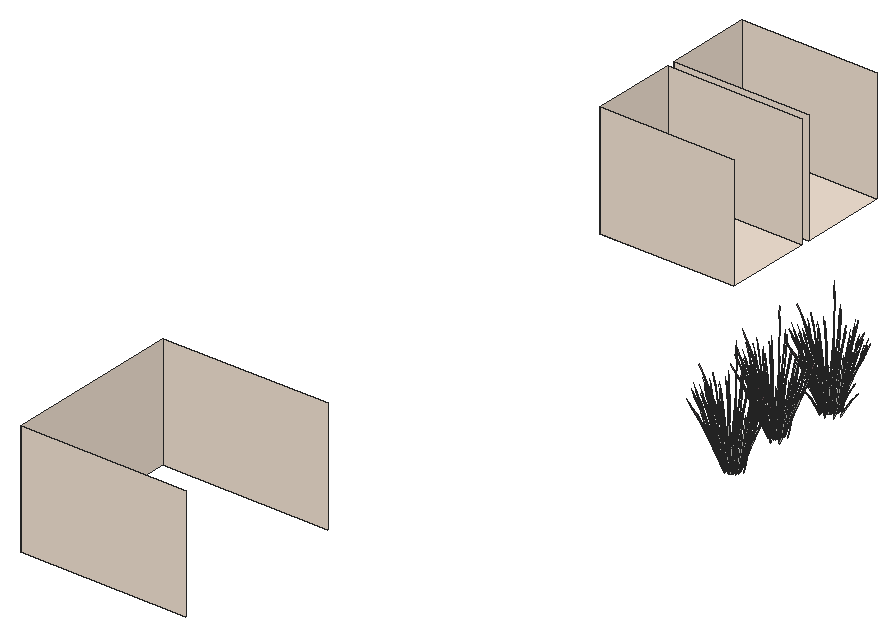
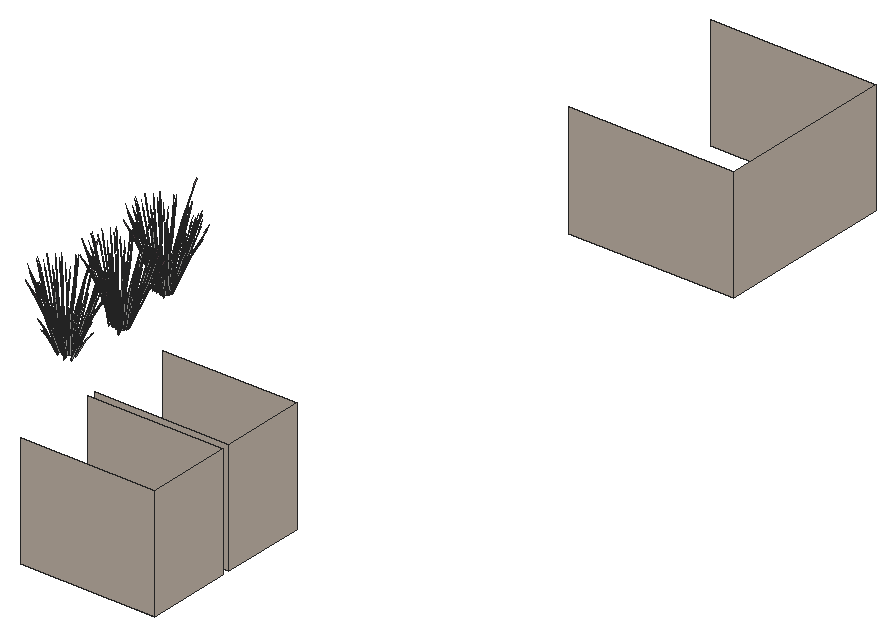
# SketchUp Ruby script. Lengths in inches.
U = 1.inch
M = Sketchup.active_model
def pt(a) = Geom::Point3d.new(a.map { |v| v * U })
def face(e, loops, mat)
  f = e.add_face(loops[0].map { |a| pt(a) })
  loops[1..].each { |l| e.add_face(l.map { |a| pt(a) }).erase! }
  f.material = f.back_material = mat if mat
  f
end
# faces: each face lists its corners as indices into pts; further lists are holes
def faces(e, pts, list, mat = nil) = list.each { |f| face(e, (f[0].is_a?(Array) ? f : [f]).map { |l| l.map { |i| pts[i] } }, mat) }
# xy, xz, yz: faces in a plane at the given z, y or x. An outline is a flat list of corners, or four numbers for a rectangle; further outlines are holes
def ring(l) = l.size == 4 ? [[l[0], l[1]], [l[2], l[1]], [l[2], l[3]], [l[0], l[3]]] : l.each_slice(2).to_a
def flat(e, list, mat, &to3) = list.each { |f| face(e, (f[0].is_a?(Array) ? f : [f]).map { |l| ring(l).map { |u, v| to3.(u, v) } }, mat) }
def xy(e, z, list, mat = nil) = flat(e, list, mat) { |x, y| [x, y, z] }
def xz(e, y, list, mat = nil) = flat(e, list, mat) { |x, z| [x, y, z] }
def yz(e, x, list, mat = nil) = flat(e, list, mat) { |y, z| [x, y, z] }
def lines(e, pts, list) = list.each { |a, b| e.add_line(pt(pts[a]), pt(pts[b])) }
# prism: a flat outline (further loops are holes) pulled along v
def prism(e, loops, v, mat = nil)
  f = face(e, loops, mat); d = Geom::Vector3d.new(v.map { |x| x * U })
  f.pushpull(f.normal.samedirection?(d) ? d.length : -d.length)
end
def box(e, o, s, mat = nil) = prism(e, [[o, [o[0] + s[0], o[1], o[2]], [o[0] + s[0], o[1] + s[1], o[2]], [o[0], o[1] + s[1], o[2]]]], [0, 0, s[2]], mat)
def at(x, y, z, deg = 0) = Geom::Transformation.translation(pt([x, y, z])) * Geom::Transformation.rotation(ORIGIN, Z_AXIS, deg.degrees)
def axes(o, x, y, z) = Geom::Transformation.new([*x, 0, *y, 0, *z, 0, *pt(o).to_a, 1])
def part(name) = M.definitions.add(name)
# library, detail: a bought-in or finely detailed component or shape, given as its bounding box
def library(name, o, s) = part(name).tap { |d| box(d.entities, o, s) }
def detail(e, o, s) = box(e.add_group.entities, o, s)
def put(e, d, t, mat = nil) = e.add_instance(d, t).tap { |i| i.material = mat if mat }
def group(e, t, mat = nil) = e.add_group.tap { |g| g.transformation = t; g.material = mat if mat }.entities
root = M.entities
M.materials.add("C01_Vanilla_Cream").color = [244, 228, 212]
M.materials.add("LightPink_Translucent").color = [144, 107, 117]
M.materials["LightPink_Translucent"].alpha = 0.75
c1 = part("blade")
p = [[2.15,0.21,22],[0,0.17,0],[0.09,0.45,0],[2.18,0.31,22],[2.29,0.31,22],[0.38,0.45,0],
  [2.48,0.24,33],[2.49,0.24,33],[2.48,0.22,33]]
faces(c1.entities,p,[[0,1,2,3],[4,5,2,3],[6,3,4,7],[8,0,3,6]])
c2 = part("seeds")
p = [[0.3,-0.1,1.38],[-0.01,-0.03,1.59],[-0.01,-0.03,0.03],[0.14,-0.07,-0.07],[0.29,-0.03,3],[0.15,0.01,3.11]]
faces(c2.entities,p,[[0,1,2,3],[1,0,4,5]],"LightPink_Translucent")
c3 = part("blade with seeds")
put(c3.entities,c1,at(0,0,0))
put(c3.entities,c2,axes([2.4,0.25,30.99],[1.5799,-0.05474,1.17369],[-0.12525,1.92788,0.29478],[-0.07173,-0.02425,1.56792]))
xy(root,501,[[240,327,290,358.5],[240,361.5,290,393]],"C01_Vanilla_Cream")
xz(root,75,[[226.53,501,288,543]],"C01_Vanilla_Cream")
xz(root,141,[[226.53,501,288,543]],"C01_Vanilla_Cream")
xz(root,327,[[240,501,290,543]],"C01_Vanilla_Cream")
xz(root,358.5,[[240,501,290,543]],"C01_Vanilla_Cream")
xz(root,361.5,[[240,501,290,543]],"C01_Vanilla_Cream")
xz(root,393,[[240,501,290,543]],"C01_Vanilla_Cream")
yz(root,226.53,[[75,501,141,543]],"C01_Vanilla_Cream")
yz(root,240,[[327,501,358.5,543],[361.5,501,393,543]],"C01_Vanilla_Cream")
put(root,c3,axes([353.4,268.07,500.07],[-0.01441,-0.29294,0.86145],[0.36003,0.20894,0.63294],[-0.07081,0.13963,0.18974]))
put(root,c3,axes([357.67,263.51,500.07],[-0.18544,0.25079,0.86145],[-0.15939,-0.33694,0.63294],[0.15316,-0.08443,0.18974]))
put(root,c3,axes([355.34,262.26,500.07],[0.07142,0.28728,0.86145],[-0.3962,-0.15911,0.63294],[0.04263,-0.1471,0.18974]))
put(root,c3,axes([354.97,286.16,500.07],[0.35544,-0.03525,0.86145],[-0.22547,0.31061,0.63294],[-0.17565,-0.04659,0.18974]))
put(root,c3,axes([359.68,288.375,500.07],[-0.31347,-0.14166,0.86145],[0.40476,-0.14393,0.63294],[0.10917,0.12192,0.18974]))
put(root,c3,axes([354.47,288.61,500.07],[0.23202,-0.22328,0.86145],[0.09155,0.35348,0.63294],[-0.16768,0.06329,0.18974]))
put(root,c3,axes([361.59,287.21,500.07],[-0.34399,0.08133,0.86145],[0.16192,-0.33614,0.63294],[0.18249,0.023,0.18974]))
put(root,c3,axes([356.34,284.13,500.07],[0.29042,0.17147,0.86145],[-0.42295,0.10307,0.63294],[-0.0905,-0.13178,0.18974]))
put(root,c3,axes([356.4375,289.59,500.07],[-0.01441,-0.29294,0.86145],[0.36003,0.20894,0.63294],[-0.07081,0.13963,0.18974]))
put(root,c3,axes([360.71,285.03,500.07],[-0.18544,0.25079,0.86145],[-0.15939,-0.33694,0.63294],[0.15316,-0.08443,0.18974]))
put(root,c3,axes([358.37,283.78,500.07],[0.07142,0.28728,0.86145],[-0.3962,-0.15911,0.63294],[0.04263,-0.1471,0.18974]))
put(root,c3,axes([358.92,241.3,500.13],[-0.01521,-0.46386,1.05954],[0.68831,0.12024,0.44862],[-0.1628,0.25382,1.00012]))
put(root,c3,axes([355.88,265.26,500.13],[-0.01521,-0.46386,1.05954],[0.68831,0.12024,0.44862],[-0.1628,0.25382,1.00012]))
put(root,c3,axes([358.92,286.78,500.13],[-0.01521,-0.46386,1.05954],[0.68831,0.12024,0.44862],[-0.1628,0.25382,1.00012]))
put(root,c3,axes([357.04,239.55,501.74],[-0.47473,-0.23813,-0.53284],[0.33738,-0.41728,0.0643],[-0.172,-0.14218,0.75375]))
put(root,c3,axes([357.55,243.21,501.74],[0.26572,0.40059,-0.53284],[-0.54698,0.22325,0.0643],[0.06214,0.19355,0.75375]))
put(root,c3,axes([356.07,240.14,501.74],[-0.55654,-0.01186,-0.53284],[0.03738,-0.49951,0.0643],[-0.23578,-0.05271,0.75375]))
put(root,c3,axes([360.06,240.62,501.74],[0.29081,-0.38873,-0.53284],[0.5096,0.27626,0.0643],[0.17364,-0.14084,0.75375]))
put(root,c3,axes([360.2,241.6,501.74],[0.48922,-0.21758,-0.53284],[0.27264,0.44789,0.0643],[0.23638,-0.05088,0.75375]))
put(root,c3,axes([359.34,239.83,501.74],[0.01449,-0.45571,-0.53284],[0.61002,0.03061,0.0643],[0.06438,-0.19306,0.75375]))
put(root,c3,axes([359.72,242.51,501.74],[0.55654,0.01186,-0.53284],[-0.03738,0.49951,0.0643],[0.23578,0.05271,0.75375]))
put(root,c3,axes([358.23,239.4375,501.74],[-0.26572,-0.40059,-0.53284],[0.54698,-0.22325,0.0643],[-0.06214,-0.19355,0.75375]))
put(root,c3,axes([354,263.52,501.74],[-0.47473,-0.23813,-0.53284],[0.33738,-0.41728,0.0643],[-0.172,-0.14218,0.75375]))
put(root,c3,axes([354.52,267.18,501.74],[0.26572,0.40059,-0.53284],[-0.54698,0.22325,0.0643],[0.06214,0.19355,0.75375]))
put(root,c3,axes([353.03,264.11,501.74],[-0.55654,-0.01186,-0.53284],[0.03738,-0.49951,0.0643],[-0.23578,-0.05271,0.75375]))
put(root,c3,axes([357.02,264.59,501.74],[0.29081,-0.38873,-0.53284],[0.5096,0.27626,0.0643],[0.17364,-0.14084,0.75375]))
put(root,c3,axes([357.16,265.57,501.74],[0.48922,-0.21758,-0.53284],[0.27264,0.44789,0.0643],[0.23638,-0.05088,0.75375]))
put(root,c3,axes([356.3,263.8,501.74],[0.01449,-0.45571,-0.53284],[0.61002,0.03061,0.0643],[0.06438,-0.19306,0.75375]))
put(root,c3,axes([356.68,266.48,501.74],[0.55654,0.01186,-0.53284],[-0.03738,0.49951,0.0643],[0.23578,0.05271,0.75375]))
put(root,c3,axes([355.2,263.4,501.74],[-0.26572,-0.40059,-0.53284],[0.54698,-0.22325,0.0643],[-0.06214,-0.19355,0.75375]))
put(root,c3,axes([357.04,285.04,501.74],[-0.47473,-0.23813,-0.53284],[0.33738,-0.41728,0.0643],[-0.172,-0.14218,0.75375]))
put(root,c3,axes([357.55,288.7,501.74],[0.26572,0.40059,-0.53284],[-0.54698,0.22325,0.0643],[0.06214,0.19355,0.75375]))
put(root,c3,axes([356.07,285.625,501.74],[-0.55654,-0.01186,-0.53284],[0.03738,-0.49951,0.0643],[-0.23578,-0.05271,0.75375]))
put(root,c3,axes([360.06,286.11,501.74],[0.29081,-0.38873,-0.53284],[0.5096,0.27626,0.0643],[0.17364,-0.14084,0.75375]))
put(root,c3,axes([360.2,287.09,501.74],[0.48922,-0.21758,-0.53284],[0.27264,0.44789,0.0643],[0.23638,-0.05088,0.75375]))
put(root,c3,axes([359.34,285.31,501.74],[0.01449,-0.45571,-0.53284],[0.61002,0.03061,0.0643],[0.06438,-0.19306,0.75375]))
put(root,c3,axes([359.72,287.99,501.74],[0.55654,0.01186,-0.53284],[-0.03738,0.49951,0.0643],[0.23578,0.05271,0.75375]))
put(root,c3,axes([358.23,284.92,501.74],[-0.26572,-0.40059,-0.53284],[0.54698,-0.22325,0.0643],[-0.06214,-0.19355,0.75375]))
put(root,c3,axes([357.75,243.29,501.51],[0.54728,0.1235,-0.38324],[-0.18759,0.42344,-0.29685],[0.05018,0.17048,0.7333]))
put(root,c3,axes([359.22,239.68,501.51],[-0.39855,-0.33102,-0.38324],[0.42102,-0.2899,-0.29685],[0.06064,-0.16819,0.7333]))
put(root,c3,axes([356.81,239.5625,501.51],[-0.54938,0.11711,-0.38324],[-0.0961,-0.44351,-0.29685],[-0.14756,-0.1271,0.7333]))
put(root,c3,axes([360.3,241.4375,501.51],[0.15083,-0.44814,-0.38324],[0.51712,0.15361,-0.29685],[0.2082,-0.04109,0.7333]))
put(root,c3,axes([355.88,240.24,501.51],[-0.40426,0.32635,-0.38324],[-0.35404,-0.34474,-0.29685],[-0.2054,-0.04965,0.7333]))
put(root,c3,axes([355.74,242.21,501.51],[0.14302,0.44985,-0.38324],[-0.54163,0.07869,-0.29685],[-0.15522,0.12083,0.7333]))
put(root,c3,axes([355.49,241.21,501.51],[-0.15083,0.44814,-0.38324],[-0.51712,-0.15361,-0.29685],[-0.2082,0.04109,0.7333]))
put(root,c3,axes([358.03,239.36,501.51],[-0.54728,-0.1235,-0.38324],[0.18759,-0.42344,-0.29685],[-0.05018,-0.17048,0.7333]))
put(root,c3,axes([360.04,240.44,501.51],[-0.14302,-0.44985,-0.38324],[0.54163,-0.07869,-0.29685],[0.15522,-0.12083,0.7333]))
put(root,c3,axes([358.97,243.09,501.51],[0.54938,-0.11711,-0.38324],[0.0961,0.44351,-0.29685],[0.14756,0.1271,0.7333]))
put(root,c3,axes([354.72,267.26,501.51],[0.54728,0.1235,-0.38324],[-0.18759,0.42344,-0.29685],[0.05018,0.17048,0.7333]))
put(root,c3,axes([356.18,263.65,501.51],[-0.39855,-0.33102,-0.38324],[0.42102,-0.2899,-0.29685],[0.06064,-0.16819,0.7333]))
put(root,c3,axes([353.78,263.53,501.51],[-0.54938,0.11711,-0.38324],[-0.0961,-0.44351,-0.29685],[-0.14756,-0.1271,0.7333]))
put(root,c3,axes([357.26,265.41,501.51],[0.15083,-0.44814,-0.38324],[0.51712,0.15361,-0.29685],[0.2082,-0.04109,0.7333]))
put(root,c3,axes([352.85,264.21,501.51],[-0.40426,0.32635,-0.38324],[-0.35404,-0.34474,-0.29685],[-0.2054,-0.04965,0.7333]))
put(root,c3,axes([352.71,266.17,501.51],[0.14302,0.44985,-0.38324],[-0.54163,0.07869,-0.29685],[-0.15522,0.12083,0.7333]))
put(root,c3,axes([352.45,265.18,501.51],[-0.15083,0.44814,-0.38324],[-0.51712,-0.15361,-0.29685],[-0.2082,0.04109,0.7333]))
put(root,c3,axes([355,263.32,501.51],[-0.54728,-0.1235,-0.38324],[0.18759,-0.42344,-0.29685],[-0.05018,-0.17048,0.7333]))
put(root,c3,axes([357.01,264.41,501.51],[-0.14302,-0.44985,-0.38324],[0.54163,-0.07869,-0.29685],[0.15522,-0.12083,0.7333]))
put(root,c3,axes([355.9375,267.05,501.51],[0.54938,-0.11711,-0.38324],[0.0961,0.44351,-0.29685],[0.14756,0.1271,0.7333]))
put(root,c3,axes([357.75,288.78,501.51],[0.54728,0.1235,-0.38324],[-0.18759,0.42344,-0.29685],[0.05018,0.17048,0.7333]))
put(root,c3,axes([359.22,285.16,501.51],[-0.39855,-0.33102,-0.38324],[0.42102,-0.2899,-0.29685],[0.06064,-0.16819,0.7333]))
put(root,c3,axes([356.81,285.05,501.51],[-0.54938,0.11711,-0.38324],[-0.0961,-0.44351,-0.29685],[-0.14756,-0.1271,0.7333]))
put(root,c3,axes([360.3,286.92,501.51],[0.15083,-0.44814,-0.38324],[0.51712,0.15361,-0.29685],[0.2082,-0.04109,0.7333]))
put(root,c3,axes([355.88,285.73,501.51],[-0.40426,0.32635,-0.38324],[-0.35404,-0.34474,-0.29685],[-0.2054,-0.04965,0.7333]))
put(root,c3,axes([355.74,287.69,501.51],[0.14302,0.44985,-0.38324],[-0.54163,0.07869,-0.29685],[-0.15522,0.12083,0.7333]))
put(root,c3,axes([355.49,286.69,501.51],[-0.15083,0.44814,-0.38324],[-0.51712,-0.15361,-0.29685],[-0.2082,0.04109,0.7333]))
put(root,c3,axes([358.03,284.84,501.51],[-0.54728,-0.1235,-0.38324],[0.18759,-0.42344,-0.29685],[-0.05018,-0.17048,0.7333]))
put(root,c3,axes([360.04,285.93,501.51],[-0.14302,-0.44985,-0.38324],[0.54163,-0.07869,-0.29685],[0.15522,-0.12083,0.7333]))
put(root,c3,axes([358.97,288.57,501.51],[0.54938,-0.11711,-0.38324],[0.0961,0.44351,-0.29685],[0.14756,0.1271,0.7333]))
put(root,c3,axes([356.45,242.82,502],[-0.01449,0.45571,-0.59145],[-0.61002,-0.03061,0.07138],[-0.06438,0.19306,0.83667]))
put(root,c3,axes([353.41,266.79,502],[-0.01449,0.45571,-0.59145],[-0.61002,-0.03061,0.07138],[-0.06438,0.19306,0.83667]))
put(root,c3,axes([356.45,288.3,502],[-0.01449,0.45571,-0.59145],[-0.61002,-0.03061,0.07138],[-0.06438,0.19306,0.83667]))
put(root,c3,axes([356.57,242.97,501.75],[0.39855,0.33102,-0.4254],[-0.42102,0.2899,-0.32951],[-0.06064,0.16819,0.81396]))
put(root,c3,axes([353.53,266.9375,501.75],[0.39855,0.33102,-0.4254],[-0.42102,0.2899,-0.32951],[-0.06064,0.16819,0.81396]))
put(root,c3,axes([356.57,288.46,501.75],[0.39855,0.33102,-0.4254],[-0.42102,0.2899,-0.32951],[-0.06064,0.16819,0.81396]))
put(root,c3,axes([358.17,242.25,500.49],[0.48111,0.19866,1.13446],[-0.47133,0.42798,0.44862],[-0.21112,-0.25366,0.95105]))
put(root,c3,axes([355.14,266.21,500.49],[0.48111,0.19866,1.13446],[-0.47133,0.42798,0.44862],[-0.21112,-0.25366,0.95105]))
put(root,c3,axes([358.17,287.73,500.49],[0.48111,0.19866,1.13446],[-0.47133,0.42798,0.44862],[-0.21112,-0.25366,0.95105]))
put(root,c3,axes([356.58,240.9375,500.51],[0.15825,-0.07127,1.32798],[0.05457,0.4976,0.10393],[-0.34278,0.06603,0.47463]))
put(root,c3,axes([353.55,264.9,500.51],[0.15825,-0.07127,1.32798],[0.05457,0.4976,0.10393],[-0.34278,0.06603,0.47463]))
put(root,c3,axes([356.58,286.42,500.51],[0.15825,-0.07127,1.32798],[0.05457,0.4976,0.10393],[-0.34278,0.06603,0.47463]))
put(root,c3,axes([356.24,243.46,500.52],[0.01223,-0.25433,1.15759],[0.55017,0.13434,0.15997],[-0.04767,0.27105,0.54661]))
put(root,c3,axes([353.21,267.43,500.52],[0.01223,-0.25433,1.15759],[0.55017,0.13434,0.15997],[-0.04767,0.27105,0.54661]))
put(root,c3,axes([356.24,288.95,500.52],[0.01223,-0.25433,1.15759],[0.55017,0.13434,0.15997],[-0.04767,0.27105,0.54661]))
put(root,c3,axes([360.05,242.71,501.39],[0.31678,0.30846,-0.2656],[-0.36171,0.29199,0.3429],[0.18378,0.04443,0.65611]))
put(root,c3,axes([355.17,241.01,501.39],[-0.46269,-0.13744,-0.2656],[0.13495,-0.40096,0.3429],[-0.18628,0.03677,0.65611]))
put(root,c3,axes([355.34,242.16,501.39],[-0.48462,0.07041,-0.2656],[-0.12797,-0.4025,0.3429],[-0.13888,0.10811,0.65611]))
put(root,c3,axes([360.61,241.64,501.39],[0.46269,0.13744,-0.2656],[-0.13495,0.40096,0.3429],[0.18628,-0.03677,0.65611]))
put(root,c3,axes([356.87,239.24,501.39],[-0.08599,-0.39682,-0.2656],[0.49155,-0.10478,0.3429],[-0.13203,-0.11372,0.65611]))
put(root,c3,axes([356.2,243.09,501.39],[-0.3767,0.25939,-0.2656],[-0.3566,-0.29618,0.3429],[-0.05426,0.15048,0.65611]))
put(root,c3,axes([360.44,240.49,501.39],[0.48462,-0.07041,-0.2656],[0.12797,0.4025,0.3429],[0.13888,-0.10811,0.65611]))
put(root,c3,axes([357.5,243.55,501.39],[-0.16784,0.37886,-0.2656],[-0.48968,-0.1105,0.3429],[0.0449,0.15254,0.65611]))
put(root,c3,axes([359.59,239.56,501.39],[0.3767,-0.25939,-0.2656],[0.3566,0.29618,0.3429],[0.05426,-0.15048,0.65611]))
put(root,c3,axes([358.28,239.1,501.39],[0.16784,-0.37886,-0.2656],[0.48968,0.1105,0.3429],[-0.0449,-0.15254,0.65611]))
put(root,c3,axes([355.73,239.93,501.39],[-0.31678,-0.30846,-0.2656],[0.36171,-0.29199,0.3429],[-0.18378,-0.04443,0.65611]))
put(root,c3,axes([357.02,266.68,501.39],[0.31678,0.30846,-0.2656],[-0.36171,0.29199,0.3429],[0.18378,0.04443,0.65611]))
put(root,c3,axes([352.14,264.97,501.39],[-0.46269,-0.13744,-0.2656],[0.13495,-0.40096,0.3429],[-0.18628,0.03677,0.65611]))
put(root,c3,axes([352.31,266.13,501.39],[-0.48462,0.07041,-0.2656],[-0.12797,-0.4025,0.3429],[-0.13888,0.10811,0.65611]))
put(root,c3,axes([357.58,265.61,501.39],[0.46269,0.13744,-0.2656],[-0.13495,0.40096,0.3429],[0.18628,-0.03677,0.65611]))
put(root,c3,axes([353.83,263.2,501.39],[-0.08599,-0.39682,-0.2656],[0.49155,-0.10478,0.3429],[-0.13203,-0.11372,0.65611]))
put(root,c3,axes([353.16,267.06,501.39],[-0.3767,0.25939,-0.2656],[-0.3566,-0.29618,0.3429],[-0.05426,0.15048,0.65611]))
put(root,c3,axes([357.41,264.45,501.39],[0.48462,-0.07041,-0.2656],[0.12797,0.4025,0.3429],[0.13888,-0.10811,0.65611]))
put(root,c3,axes([354.47,267.52,501.39],[-0.16784,0.37886,-0.2656],[-0.48968,-0.1105,0.3429],[0.0449,0.15254,0.65611]))
put(root,c3,axes([356.55,263.52,501.39],[0.3767,-0.25939,-0.2656],[0.3566,0.29618,0.3429],[0.05426,-0.15048,0.65611]))
put(root,c3,axes([355.25,263.0625,501.39],[0.16784,-0.37886,-0.2656],[0.48968,0.1105,0.3429],[-0.0449,-0.15254,0.65611]))
put(root,c3,axes([352.7,263.9,501.39],[-0.31678,-0.30846,-0.2656],[0.36171,-0.29199,0.3429],[-0.18378,-0.04443,0.65611]))
put(root,c3,axes([360.05,288.2,501.39],[0.31678,0.30846,-0.2656],[-0.36171,0.29199,0.3429],[0.18378,0.04443,0.65611]))
put(root,c3,axes([355.17,286.49,501.39],[-0.46269,-0.13744,-0.2656],[0.13495,-0.40096,0.3429],[-0.18628,0.03677,0.65611]))
put(root,c3,axes([355.34,287.65,501.39],[-0.48462,0.07041,-0.2656],[-0.12797,-0.4025,0.3429],[-0.13888,0.10811,0.65611]))
put(root,c3,axes([360.61,287.13,501.39],[0.46269,0.13744,-0.2656],[-0.13495,0.40096,0.3429],[0.18628,-0.03677,0.65611]))
put(root,c3,axes([356.87,284.72,501.39],[-0.08599,-0.39682,-0.2656],[0.49155,-0.10478,0.3429],[-0.13203,-0.11372,0.65611]))
put(root,c3,axes([356.2,288.58,501.39],[-0.3767,0.25939,-0.2656],[-0.3566,-0.29618,0.3429],[-0.05426,0.15048,0.65611]))
put(root,c3,axes([360.44,285.97,501.39],[0.48462,-0.07041,-0.2656],[0.12797,0.4025,0.3429],[0.13888,-0.10811,0.65611]))
put(root,c3,axes([357.5,289.04,501.39],[-0.16784,0.37886,-0.2656],[-0.48968,-0.1105,0.3429],[0.0449,0.15254,0.65611]))
put(root,c3,axes([359.59,285.04,501.39],[0.3767,-0.25939,-0.2656],[0.3566,0.29618,0.3429],[0.05426,-0.15048,0.65611]))
put(root,c3,axes([358.28,284.58,501.39],[0.16784,-0.37886,-0.2656],[0.48968,0.1105,0.3429],[-0.0449,-0.15254,0.65611]))
put(root,c3,axes([355.73,285.42,501.39],[-0.31678,-0.30846,-0.2656],[0.36171,-0.29199,0.3429],[-0.18378,-0.04443,0.65611]))
put(root,c3,axes([361,242.76,500.95],[-0.10656,-0.41414,-0.02619],[0.50364,-0.09521,-0.11874],[0.10517,0.02626,0.39164]))
put(root,c3,axes([357.96,266.73,500.95],[-0.10656,-0.41414,-0.02619],[0.50364,-0.09521,-0.11874],[0.10517,0.02626,0.39164]))
put(root,c3,axes([361,288.25,500.95],[-0.10656,-0.41414,-0.02619],[0.50364,-0.09521,-0.11874],[0.10517,0.02626,0.39164]))
put(root,c3,axes([358.92,241.92,500.91],[-0.2068,-0.08488,1.28532],[0.42797,-0.35609,0.10393],[0.26673,0.16064,0.54946]))
put(root,c3,axes([358.65,239.6,500.91],[-0.10366,0.16934,1.28532],[-0.43488,-0.35044,0.10393],[0.19618,-0.21841,0.54946]))
put(root,c3,axes([359.35,241.15,500.91],[-0.23093,0.01116,1.28532],[0.15319,-0.4836,0.10393],[0.32909,0.02991,0.54946]))
put(root,c3,axes([358.0625,242.42,500.91],[-0.12726,-0.15818,1.28532],[0.58807,-0.13317,0.10393],[0.13291,0.24832,0.54946]))
put(root,c3,axes([357.02,242.5,500.91],[-0.01363,-0.18909,1.28532],[0.5906,0.12544,0.10393],[-0.03653,0.26947,0.54946]))
put(root,c3,axes([356.08,242.14,500.91],[0.10366,-0.16934,1.28532],[0.43488,0.35044,0.10393],[-0.19618,0.21841,0.54946]))
put(root,c3,axes([355.47,241.44,500.91],[0.19317,-0.10421,1.28532],[0.16263,0.48153,0.10393],[-0.30326,0.10883,0.54946]))
put(root,c3,axes([356.18,241.77,500.91],[0.13906,-0.15138,1.28532],[0.35111,0.40859,0.10393],[-0.24082,0.18608,0.54946]))
put(root,c3,axes([356.67,239.32,500.91],[0.12726,0.15818,1.28532],[-0.58807,0.13317,0.10393],[-0.13291,-0.24832,0.54946]))
put(root,c3,axes([355.81,239.8125,500.91],[0.2068,0.08488,1.28532],[-0.42797,0.35609,0.10393],[-0.26673,-0.16064,0.54946]))
put(root,c3,axes([355.38,240.59,500.91],[0.23093,-0.01116,1.28532],[-0.15319,0.4836,0.10393],[-0.32909,-0.02991,0.54946]))
put(root,c3,axes([355.88,265.89,500.91],[-0.2068,-0.08488,1.28532],[0.42797,-0.35609,0.10393],[0.26673,0.16064,0.54946]))
put(root,c3,axes([355.62,263.57,500.91],[-0.10366,0.16934,1.28532],[-0.43488,-0.35044,0.10393],[0.19618,-0.21841,0.54946]))
put(root,c3,axes([356.31,265.11,500.91],[-0.23093,0.01116,1.28532],[0.15319,-0.4836,0.10393],[0.32909,0.02991,0.54946]))
put(root,c3,axes([355.03,266.38,500.91],[-0.12726,-0.15818,1.28532],[0.58807,-0.13317,0.10393],[0.13291,0.24832,0.54946]))
put(root,c3,axes([353.99,266.46,500.91],[-0.01363,-0.18909,1.28532],[0.5906,0.12544,0.10393],[-0.03653,0.26947,0.54946]))
put(root,c3,axes([353.04,266.1,500.91],[0.10366,-0.16934,1.28532],[0.43488,0.35044,0.10393],[-0.19618,0.21841,0.54946]))
put(root,c3,axes([352.4375,265.41,500.91],[0.19317,-0.10421,1.28532],[0.16263,0.48153,0.10393],[-0.30326,0.10883,0.54946]))
put(root,c3,axes([353.14,265.73,500.91],[0.13906,-0.15138,1.28532],[0.35111,0.40859,0.10393],[-0.24082,0.18608,0.54946]))
put(root,c3,axes([353.63,263.29,500.91],[0.12726,0.15818,1.28532],[-0.58807,0.13317,0.10393],[-0.13291,-0.24832,0.54946]))
put(root,c3,axes([352.78,263.78,500.91],[0.2068,0.08488,1.28532],[-0.42797,0.35609,0.10393],[-0.26673,-0.16064,0.54946]))
put(root,c3,axes([352.34,264.56,500.91],[0.23093,-0.01116,1.28532],[-0.15319,0.4836,0.10393],[-0.32909,-0.02991,0.54946]))
put(root,c3,axes([358.92,287.41,500.91],[-0.2068,-0.08488,1.28532],[0.42797,-0.35609,0.10393],[0.26673,0.16064,0.54946]))
put(root,c3,axes([358.65,285.08,500.91],[-0.10366,0.16934,1.28532],[-0.43488,-0.35044,0.10393],[0.19618,-0.21841,0.54946]))
put(root,c3,axes([359.35,286.63,500.91],[-0.23093,0.01116,1.28532],[0.15319,-0.4836,0.10393],[0.32909,0.02991,0.54946]))
put(root,c3,axes([358.0625,287.9,500.91],[-0.12726,-0.15818,1.28532],[0.58807,-0.13317,0.10393],[0.13291,0.24832,0.54946]))
put(root,c3,axes([357.02,287.98,500.91],[-0.01363,-0.18909,1.28532],[0.5906,0.12544,0.10393],[-0.03653,0.26947,0.54946]))
put(root,c3,axes([356.08,287.625,500.91],[0.10366,-0.16934,1.28532],[0.43488,0.35044,0.10393],[-0.19618,0.21841,0.54946]))
put(root,c3,axes([355.47,286.93,500.91],[0.19317,-0.10421,1.28532],[0.16263,0.48153,0.10393],[-0.30326,0.10883,0.54946]))
put(root,c3,axes([356.18,287.25,500.91],[0.13906,-0.15138,1.28532],[0.35111,0.40859,0.10393],[-0.24082,0.18608,0.54946]))
put(root,c3,axes([356.67,284.81,500.91],[0.12726,0.15818,1.28532],[-0.58807,0.13317,0.10393],[-0.13291,-0.24832,0.54946]))
put(root,c3,axes([355.81,285.3,500.91],[0.2068,0.08488,1.28532],[-0.42797,0.35609,0.10393],[-0.26673,-0.16064,0.54946]))
put(root,c3,axes([355.38,286.07,500.91],[0.23093,-0.01116,1.28532],[-0.15319,0.4836,0.10393],[-0.32909,-0.02991,0.54946]))
put(root,c3,axes([359.69,242.75,501.78],[0.02981,-0.50103,-0.0912],[0.56442,0.01369,-0.50621],[0.21738,0.0348,0.76918]))
put(root,c3,axes([355.47,240.83,501.78],[0.28012,0.44611,-0.0912],[-0.49717,0.21923,-0.50621],[-0.20951,0.05886,0.76918]))
put(root,c3,axes([359.63,239.85,501.78],[-0.61188,-0.02441,-0.0912],[0.01672,-0.46217,-0.50621],[0.0425,-0.178,0.76918]))
put(root,c3,axes([360.32,241.82,501.78],[-0.28012,-0.44611,-0.0912],[0.49717,-0.21923,-0.50621],[0.20951,-0.05886,0.76918]))
put(root,c3,axes([357.29,243.3125,501.78],[0.54481,-0.22937,-0.0912],[0.26773,0.4071,-0.50621],[0.07188,0.17155,0.76918]))
put(root,c3,axes([356.1,239.9,501.78],[-0.02981,0.50103,-0.0912],[-0.56442,-0.01369,-0.50621],[-0.21738,-0.0348,0.76918]))
put(root,c3,axes([358.58,243.29,501.78],[0.33176,-0.4217,-0.0912],[0.48044,0.24295,-0.50621],[0.16701,0.11914,0.76918]))
put(root,c3,axes([355.49,241.89,501.78],[0.515,0.27165,-0.0912],[-0.2967,0.3934,-0.50621],[-0.1455,0.13675,0.76918]))
put(root,c3,axes([358.5,239.34,501.78],[-0.54481,0.22937,-0.0912],[-0.26773,-0.4071,-0.50621],[-0.07188,-0.17155,0.76918]))
put(root,c3,axes([360.3,240.76,501.78],[-0.515,-0.27165,-0.0912],[0.2967,-0.3934,-0.50621],[0.1455,-0.13675,0.76918]))
put(root,c3,axes([356.65,266.72,501.78],[0.02981,-0.50103,-0.0912],[0.56442,0.01369,-0.50621],[0.21738,0.0348,0.76918]))
put(root,c3,axes([352.43,264.79,501.78],[0.28012,0.44611,-0.0912],[-0.49717,0.21923,-0.50621],[-0.20951,0.05886,0.76918]))
put(root,c3,axes([356.6,263.82,501.78],[-0.61188,-0.02441,-0.0912],[0.01672,-0.46217,-0.50621],[0.0425,-0.178,0.76918]))
put(root,c3,axes([357.28,265.79,501.78],[-0.28012,-0.44611,-0.0912],[0.49717,-0.21923,-0.50621],[0.20951,-0.05886,0.76918]))
put(root,c3,axes([354.25,267.28,501.78],[0.54481,-0.22937,-0.0912],[0.26773,0.4071,-0.50621],[0.07188,0.17155,0.76918]))
put(root,c3,axes([353.06,263.87,501.78],[-0.02981,0.50103,-0.0912],[-0.56442,-0.01369,-0.50621],[-0.21738,-0.0348,0.76918]))
put(root,c3,axes([355.54,267.26,501.78],[0.33176,-0.4217,-0.0912],[0.48044,0.24295,-0.50621],[0.16701,0.11914,0.76918]))
put(root,c3,axes([352.45,265.85,501.78],[0.515,0.27165,-0.0912],[-0.2967,0.3934,-0.50621],[-0.1455,0.13675,0.76918]))
put(root,c3,axes([355.46,263.3,501.78],[-0.54481,0.22937,-0.0912],[-0.26773,-0.4071,-0.50621],[-0.07188,-0.17155,0.76918]))
put(root,c3,axes([357.26,264.73,501.78],[-0.515,-0.27165,-0.0912],[0.2967,-0.3934,-0.50621],[0.1455,-0.13675,0.76918]))
put(root,c3,axes([359.69,288.23,501.78],[0.02981,-0.50103,-0.0912],[0.56442,0.01369,-0.50621],[0.21738,0.0348,0.76918]))
put(root,c3,axes([355.47,286.3125,501.78],[0.28012,0.44611,-0.0912],[-0.49717,0.21923,-0.50621],[-0.20951,0.05886,0.76918]))
put(root,c3,axes([359.63,285.34,501.78],[-0.61188,-0.02441,-0.0912],[0.01672,-0.46217,-0.50621],[0.0425,-0.178,0.76918]))
put(root,c3,axes([360.32,287.31,501.78],[-0.28012,-0.44611,-0.0912],[0.49717,-0.21923,-0.50621],[0.20951,-0.05886,0.76918]))
put(root,c3,axes([357.29,288.8,501.78],[0.54481,-0.22937,-0.0912],[0.26773,0.4071,-0.50621],[0.07188,0.17155,0.76918]))
